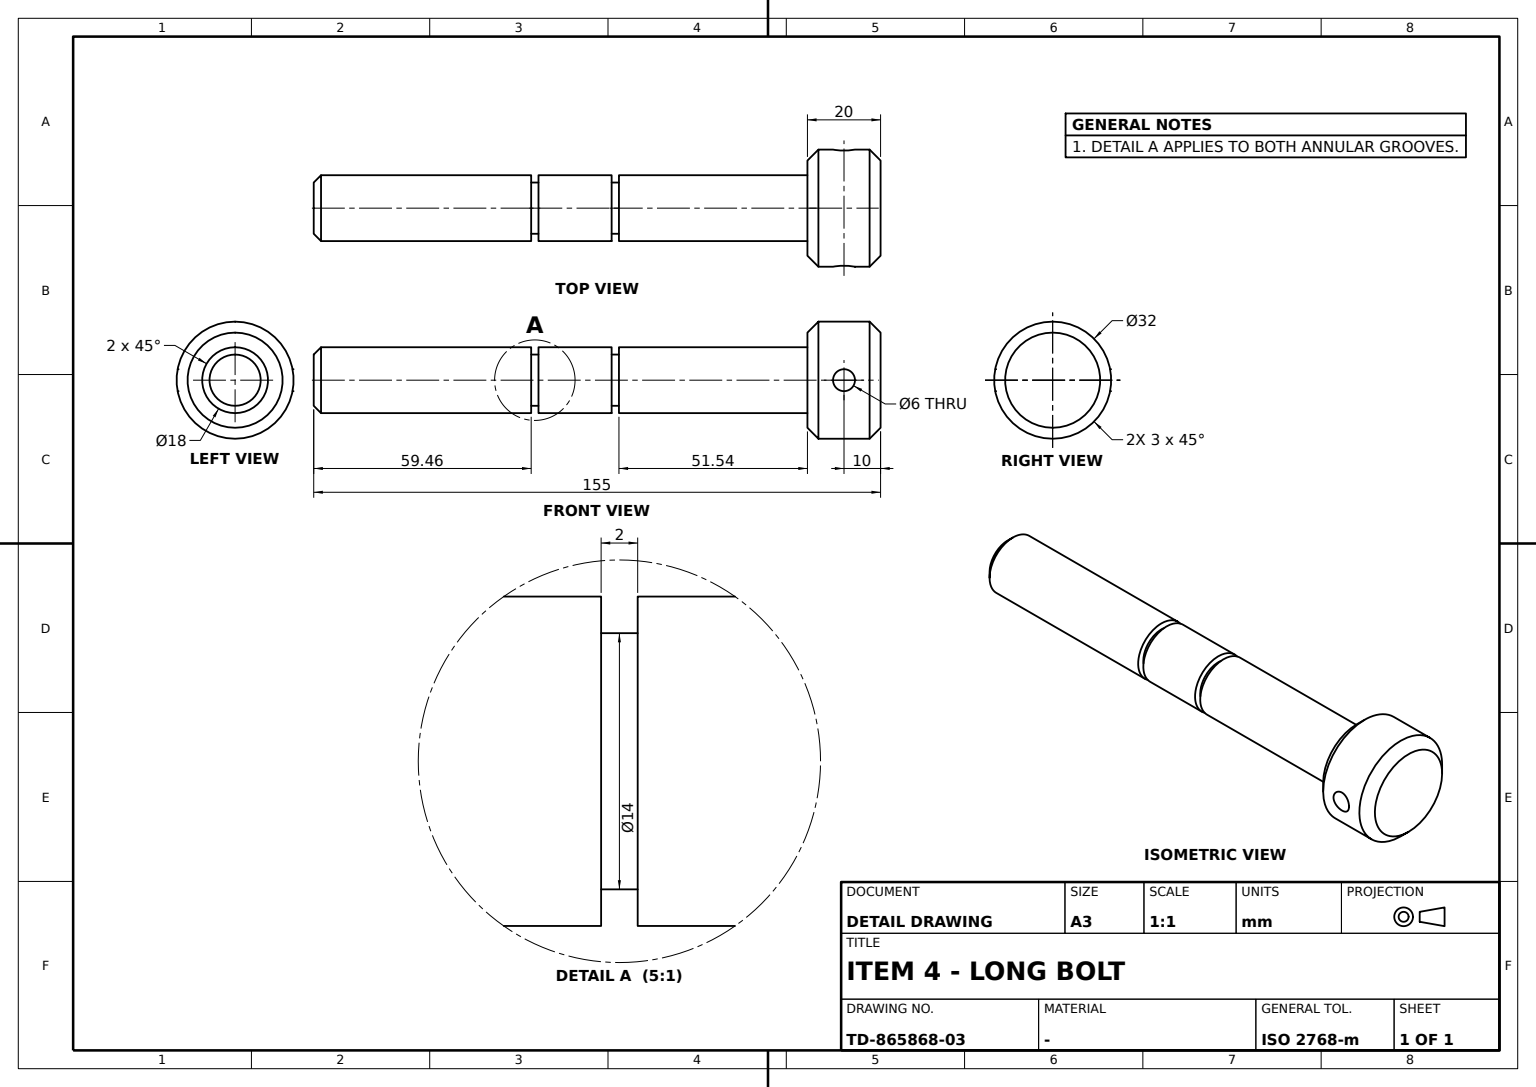
ISO-10303-21;
HEADER;
FILE_DESCRIPTION((''),'2;1');
FILE_NAME('','',(''),(''),'','','');
FILE_SCHEMA(('AUTOMOTIVE_DESIGN'));
ENDSEC;
DATA;
#1=APPLICATION_CONTEXT('');
#2=PRODUCT_CONTEXT('',#1,'mechanical');
#3=PRODUCT('','','',(#2));
#4=PRODUCT_DEFINITION_FORMATION('','',#3);
#5=PRODUCT_DEFINITION_CONTEXT('',#1,'design');
#6=PRODUCT_DEFINITION('','',#4,#5);
#7=PRODUCT_DEFINITION_SHAPE('','',#6);
#8=(LENGTH_UNIT()NAMED_UNIT(*)SI_UNIT(.MILLI.,.METRE.));
#9=(NAMED_UNIT(*)PLANE_ANGLE_UNIT()SI_UNIT($,.RADIAN.));
#10=(NAMED_UNIT(*)SI_UNIT($,.STERADIAN.)SOLID_ANGLE_UNIT());
#11=UNCERTAINTY_MEASURE_WITH_UNIT(LENGTH_MEASURE(0.005),#8,'distance_accuracy_value','');
#12=(GEOMETRIC_REPRESENTATION_CONTEXT(3)GLOBAL_UNCERTAINTY_ASSIGNED_CONTEXT((#11))GLOBAL_UNIT_ASSIGNED_CONTEXT((#8,#9,#10))REPRESENTATION_CONTEXT('',''));
#13=CARTESIAN_POINT('',(0.,81.46,-7.));
#14=VERTEX_POINT('',#13);
#15=CARTESIAN_POINT('',(0.,81.46,0.));
#16=DIRECTION('',(0.,-1.,0.));
#17=DIRECTION('',(0.,0.,-1.));
#18=AXIS2_PLACEMENT_3D('',#15,#16,#17);
#19=CIRCLE('',#18,7.);
#20=EDGE_CURVE('',#14,#14,#19,.T.);
#21=ORIENTED_EDGE('',*,*,#20,.T.);
#22=EDGE_LOOP('',(#21));
#23=FACE_BOUND('',#22,.T.);
#24=CARTESIAN_POINT('',(0.,81.46,-9.));
#25=VERTEX_POINT('',#24);
#26=CIRCLE('',#18,9.);
#27=EDGE_CURVE('',#25,#25,#26,.T.);
#28=ORIENTED_EDGE('',*,*,#27,.F.);
#29=EDGE_LOOP('',(#28));
#30=FACE_BOUND('',#29,.T.);
#31=DIRECTION('',(1.,0.,0.));
#32=AXIS2_PLACEMENT_3D('',#13,#16,#31);
#33=PLANE('',#32);
#34=ADVANCED_FACE('',(#23,#30),#33,.F.);
#35=CARTESIAN_POINT('',(0.,0.,-7.));
#36=VERTEX_POINT('',#35);
#37=CARTESIAN_POINT('',(0.,0.,0.));
#38=AXIS2_PLACEMENT_3D('',#37,#16,#17);
#39=CIRCLE('',#38,7.);
#40=EDGE_CURVE('',#36,#36,#39,.T.);
#41=ORIENTED_EDGE('',*,*,#40,.T.);
#42=EDGE_LOOP('',(#41));
#43=FACE_BOUND('',#42,.T.);
#44=CARTESIAN_POINT('',(0.,0.,-9.));
#45=AXIS2_PLACEMENT_3D('',#44,#16,#31);
#46=PLANE('',#45);
#47=ADVANCED_FACE('',(#43),#46,.T.);
#48=CARTESIAN_POINT('',(0.,2.,9.));
#49=VERTEX_POINT('',#48);
#50=CARTESIAN_POINT('',(0.,2.,0.));
#51=DIRECTION('',(0.,1.,0.));
#52=DIRECTION('',(0.,0.,1.));
#53=AXIS2_PLACEMENT_3D('',#50,#51,#52);
#54=CIRCLE('',#53,9.);
#55=EDGE_CURVE('',#49,#49,#54,.F.);
#56=ORIENTED_EDGE('',*,*,#55,.F.);
#57=EDGE_LOOP('',(#56));
#58=FACE_BOUND('',#57,.T.);
#59=CARTESIAN_POINT('',(0.,59.46,-9.));
#60=VERTEX_POINT('',#59);
#61=CARTESIAN_POINT('',(0.,59.46,0.));
#62=AXIS2_PLACEMENT_3D('',#61,#16,#17);
#63=CIRCLE('',#62,9.);
#64=EDGE_CURVE('',#60,#60,#63,.T.);
#65=ORIENTED_EDGE('',*,*,#64,.T.);
#66=EDGE_LOOP('',(#65));
#67=FACE_BOUND('',#66,.T.);
#68=CARTESIAN_POINT('',(0.,77.5,0.));
#69=AXIS2_PLACEMENT_3D('',#68,#16,#31);
#70=CYLINDRICAL_SURFACE('',#69,9.);
#71=ADVANCED_FACE('',(#58,#67),#70,.T.);
#72=CARTESIAN_POINT('',(-16.,142.,0.));
#73=VERTEX_POINT('',#72);
#74=CARTESIAN_POINT('',(-15.8591,142.650216,2.352915));
#75=CARTESIAN_POINT('',(-16.070393,141.674865,-0.000488));
#76=CARTESIAN_POINT('',(-15.859328,142.650322,-2.350963));
#77=CARTESIAN_POINT('',(-15.644744,144.996368,-3.324028));
#78=CARTESIAN_POINT('',(-15.859098,147.349771,-2.35292));
#79=CARTESIAN_POINT('',(-16.070393,148.325135,0.000455));
#80=CARTESIAN_POINT('',(-15.85933,147.34969,2.350958));
#81=CARTESIAN_POINT('',(-15.644743,145.003632,3.32403));
#82=B_SPLINE_CURVE_WITH_KNOTS('',3,(#74,#75,#76,#77,#78,#79,#80,#81,#74,#75,#76),.UNSPECIFIED.,.T.,.F.,(1,1,1,1,1,1,1,1,1,1,1,1,1,1,1),(-0.007048284,-0.004698856,-0.002349428,0.,0.002349428,0.004698856,0.007048284,0.009397711,0.011747139,0.014096567,0.016445995,0.018795423,0.021144851,0.023494278,0.025843706),.UNSPECIFIED.);
#83=EDGE_CURVE('',#73,#73,#82,.F.);
#84=ORIENTED_EDGE('',*,*,#83,.F.);
#85=EDGE_LOOP('',(#84));
#86=FACE_BOUND('',#85,.T.);
#87=CARTESIAN_POINT('',(0.,138.,16.));
#88=VERTEX_POINT('',#87);
#89=CARTESIAN_POINT('',(0.,138.,0.));
#90=AXIS2_PLACEMENT_3D('',#89,#51,#52);
#91=CIRCLE('',#90,16.);
#92=EDGE_CURVE('',#88,#88,#91,.F.);
#93=ORIENTED_EDGE('',*,*,#92,.F.);
#94=EDGE_LOOP('',(#93));
#95=FACE_BOUND('',#94,.T.);
#96=CARTESIAN_POINT('',(0.,152.,-16.));
#97=VERTEX_POINT('',#96);
#98=CARTESIAN_POINT('',(0.,152.,0.));
#99=AXIS2_PLACEMENT_3D('',#98,#16,#17);
#100=CIRCLE('',#99,16.);
#101=EDGE_CURVE('',#97,#97,#100,.T.);
#102=ORIENTED_EDGE('',*,*,#101,.T.);
#103=EDGE_LOOP('',(#102));
#104=FACE_BOUND('',#103,.T.);
#105=CARTESIAN_POINT('',(16.,148.,0.));
#106=VERTEX_POINT('',#105);
#107=CARTESIAN_POINT('',(15.8591,147.349784,-2.352915));
#108=CARTESIAN_POINT('',(16.070393,148.325135,0.000488));
#109=CARTESIAN_POINT('',(15.859328,147.349678,2.350963));
#110=CARTESIAN_POINT('',(15.644744,145.003632,3.324028));
#111=CARTESIAN_POINT('',(15.859098,142.650229,2.35292));
#112=CARTESIAN_POINT('',(16.070393,141.674865,-0.000455));
#113=CARTESIAN_POINT('',(15.85933,142.65031,-2.350958));
#114=CARTESIAN_POINT('',(15.644743,144.996368,-3.32403));
#115=B_SPLINE_CURVE_WITH_KNOTS('',3,(#107,#108,#109,#110,#111,#112,#113,#114,#107,#108,#109),.UNSPECIFIED.,.T.,.F.,(1,1,1,1,1,1,1,1,1,1,1,1,1,1,1),(-0.007048284,-0.004698856,-0.002349428,0.,0.002349428,0.004698856,0.007048284,0.009397711,0.011747139,0.014096567,0.016445995,0.018795423,0.021144851,0.023494278,0.025843706),.UNSPECIFIED.);
#116=EDGE_CURVE('',#106,#106,#115,.T.);
#117=ORIENTED_EDGE('',*,*,#116,.F.);
#118=EDGE_LOOP('',(#117));
#119=FACE_BOUND('',#118,.T.);
#120=CYLINDRICAL_SURFACE('',#69,16.);
#121=ADVANCED_FACE('',(#86,#95,#104,#119),#120,.T.);
#122=ORIENTED_EDGE('',*,*,#116,.T.);
#123=EDGE_LOOP('',(#122));
#124=FACE_BOUND('',#123,.T.);
#125=ORIENTED_EDGE('',*,*,#83,.T.);
#126=EDGE_LOOP('',(#125));
#127=FACE_BOUND('',#126,.T.);
#128=CARTESIAN_POINT('',(0.,145.,0.));
#129=AXIS2_PLACEMENT_3D('',#128,#31,#51);
#130=CYLINDRICAL_SURFACE('',#129,3.);
#131=ADVANCED_FACE('',(#124,#127),#130,.F.);
#132=ORIENTED_EDGE('',*,*,#64,.F.);
#133=EDGE_LOOP('',(#132));
#134=FACE_BOUND('',#133,.T.);
#135=CARTESIAN_POINT('',(0.,59.46,-7.));
#136=VERTEX_POINT('',#135);
#137=CIRCLE('',#62,7.);
#138=EDGE_CURVE('',#136,#136,#137,.T.);
#139=ORIENTED_EDGE('',*,*,#138,.T.);
#140=EDGE_LOOP('',(#139));
#141=FACE_BOUND('',#140,.T.);
#142=AXIS2_PLACEMENT_3D('',#135,#16,#31);
#143=PLANE('',#142);
#144=ADVANCED_FACE('',(#134,#141),#143,.F.);
#145=CARTESIAN_POINT('',(0.,61.46,-9.));
#146=VERTEX_POINT('',#145);
#147=CARTESIAN_POINT('',(0.,61.46,0.));
#148=AXIS2_PLACEMENT_3D('',#147,#16,#17);
#149=CIRCLE('',#148,9.);
#150=EDGE_CURVE('',#146,#146,#149,.T.);
#151=ORIENTED_EDGE('',*,*,#150,.T.);
#152=EDGE_LOOP('',(#151));
#153=FACE_BOUND('',#152,.T.);
#154=CARTESIAN_POINT('',(0.,61.46,-7.));
#155=VERTEX_POINT('',#154);
#156=CIRCLE('',#148,7.);
#157=EDGE_CURVE('',#155,#155,#156,.T.);
#158=ORIENTED_EDGE('',*,*,#157,.F.);
#159=EDGE_LOOP('',(#158));
#160=FACE_BOUND('',#159,.T.);
#161=AXIS2_PLACEMENT_3D('',#145,#16,#31);
#162=PLANE('',#161);
#163=ADVANCED_FACE('',(#153,#160),#162,.T.);
#164=CARTESIAN_POINT('',(0.,155.,-13.));
#165=VERTEX_POINT('',#164);
#166=CARTESIAN_POINT('',(0.,155.,0.));
#167=AXIS2_PLACEMENT_3D('',#166,#16,#17);
#168=CIRCLE('',#167,13.);
#169=EDGE_CURVE('',#165,#165,#168,.T.);
#170=ORIENTED_EDGE('',*,*,#169,.F.);
#171=EDGE_LOOP('',(#170));
#172=FACE_BOUND('',#171,.T.);
#173=AXIS2_PLACEMENT_3D('',#166,#16,#31);
#174=PLANE('',#173);
#175=ADVANCED_FACE('',(#172),#174,.F.);
#176=CARTESIAN_POINT('',(0.,83.46,-7.));
#177=VERTEX_POINT('',#176);
#178=CARTESIAN_POINT('',(0.,83.46,0.));
#179=AXIS2_PLACEMENT_3D('',#178,#16,#17);
#180=CIRCLE('',#179,7.);
#181=EDGE_CURVE('',#177,#177,#180,.T.);
#182=ORIENTED_EDGE('',*,*,#181,.T.);
#183=EDGE_LOOP('',(#182));
#184=FACE_BOUND('',#183,.T.);
#185=ORIENTED_EDGE('',*,*,#20,.F.);
#186=EDGE_LOOP('',(#185));
#187=FACE_BOUND('',#186,.T.);
#188=CYLINDRICAL_SURFACE('',#69,7.);
#189=ADVANCED_FACE('',(#184,#187),#188,.T.);
#190=ORIENTED_EDGE('',*,*,#138,.F.);
#191=EDGE_LOOP('',(#190));
#192=FACE_BOUND('',#191,.T.);
#193=ORIENTED_EDGE('',*,*,#157,.T.);
#194=EDGE_LOOP('',(#193));
#195=FACE_BOUND('',#194,.T.);
#196=ADVANCED_FACE('',(#192,#195),#188,.T.);
#197=ORIENTED_EDGE('',*,*,#27,.T.);
#198=EDGE_LOOP('',(#197));
#199=FACE_BOUND('',#198,.T.);
#200=ORIENTED_EDGE('',*,*,#150,.F.);
#201=EDGE_LOOP('',(#200));
#202=FACE_BOUND('',#201,.T.);
#203=ADVANCED_FACE('',(#199,#202),#70,.T.);
#204=CARTESIAN_POINT('',(0.,135.,-13.));
#205=VERTEX_POINT('',#204);
#206=CARTESIAN_POINT('',(0.,135.,0.));
#207=AXIS2_PLACEMENT_3D('',#206,#16,#17);
#208=CIRCLE('',#207,13.);
#209=EDGE_CURVE('',#205,#205,#208,.T.);
#210=ORIENTED_EDGE('',*,*,#209,.T.);
#211=EDGE_LOOP('',(#210));
#212=FACE_BOUND('',#211,.T.);
#213=CARTESIAN_POINT('',(0.,135.,-9.));
#214=VERTEX_POINT('',#213);
#215=CIRCLE('',#207,9.);
#216=EDGE_CURVE('',#214,#214,#215,.T.);
#217=ORIENTED_EDGE('',*,*,#216,.F.);
#218=EDGE_LOOP('',(#217));
#219=FACE_BOUND('',#218,.T.);
#220=CARTESIAN_POINT('',(0.,135.,-16.));
#221=AXIS2_PLACEMENT_3D('',#220,#16,#31);
#222=PLANE('',#221);
#223=ADVANCED_FACE('',(#212,#219),#222,.T.);
#224=ORIENTED_EDGE('',*,*,#101,.F.);
#225=EDGE_LOOP('',(#224));
#226=FACE_BOUND('',#225,.T.);
#227=ORIENTED_EDGE('',*,*,#169,.T.);
#228=EDGE_LOOP('',(#227));
#229=FACE_BOUND('',#228,.T.);
#230=CARTESIAN_POINT('',(0.,168.,0.));
#231=DIRECTION('',(0.479425539,0.,-0.877582562));
#232=AXIS2_PLACEMENT_3D('',#230,#16,#231);
#233=CONICAL_SURFACE('',#232,0.,0.785398163);
#234=ADVANCED_FACE('',(#226,#229),#233,.T.);
#235=ORIENTED_EDGE('',*,*,#55,.T.);
#236=EDGE_LOOP('',(#235));
#237=FACE_BOUND('',#236,.T.);
#238=ORIENTED_EDGE('',*,*,#40,.F.);
#239=EDGE_LOOP('',(#238));
#240=FACE_BOUND('',#239,.T.);
#241=CARTESIAN_POINT('',(0.,-7.,0.));
#242=DIRECTION('',(-0.479425539,0.,0.877582562));
#243=AXIS2_PLACEMENT_3D('',#241,#51,#242);
#244=CONICAL_SURFACE('',#243,0.,0.785398163);
#245=ADVANCED_FACE('',(#237,#240),#244,.T.);
#246=CARTESIAN_POINT('',(0.,83.46,-9.));
#247=VERTEX_POINT('',#246);
#248=CIRCLE('',#179,9.);
#249=EDGE_CURVE('',#247,#247,#248,.T.);
#250=ORIENTED_EDGE('',*,*,#249,.T.);
#251=EDGE_LOOP('',(#250));
#252=FACE_BOUND('',#251,.T.);
#253=ORIENTED_EDGE('',*,*,#181,.F.);
#254=EDGE_LOOP('',(#253));
#255=FACE_BOUND('',#254,.T.);
#256=AXIS2_PLACEMENT_3D('',#246,#16,#31);
#257=PLANE('',#256);
#258=ADVANCED_FACE('',(#252,#255),#257,.T.);
#259=ORIENTED_EDGE('',*,*,#92,.T.);
#260=EDGE_LOOP('',(#259));
#261=FACE_BOUND('',#260,.T.);
#262=ORIENTED_EDGE('',*,*,#209,.F.);
#263=EDGE_LOOP('',(#262));
#264=FACE_BOUND('',#263,.T.);
#265=CARTESIAN_POINT('',(0.,122.,0.));
#266=AXIS2_PLACEMENT_3D('',#265,#51,#242);
#267=CONICAL_SURFACE('',#266,0.,0.785398163);
#268=ADVANCED_FACE('',(#261,#264),#267,.T.);
#269=ORIENTED_EDGE('',*,*,#216,.T.);
#270=EDGE_LOOP('',(#269));
#271=FACE_BOUND('',#270,.T.);
#272=ORIENTED_EDGE('',*,*,#249,.F.);
#273=EDGE_LOOP('',(#272));
#274=FACE_BOUND('',#273,.T.);
#275=ADVANCED_FACE('',(#271,#274),#70,.T.);
#276=CLOSED_SHELL('',(#34,#47,#71,#121,#131,#144,#163,#175,#189,#196,#203,#223,#234,#245,#258,#268,#275));
#277=MANIFOLD_SOLID_BREP('',#276);
#278=ADVANCED_BREP_SHAPE_REPRESENTATION('',(#277),#12);
#279=SHAPE_DEFINITION_REPRESENTATION(#7,#278);
ENDSEC;
END-ISO-10303-21;
